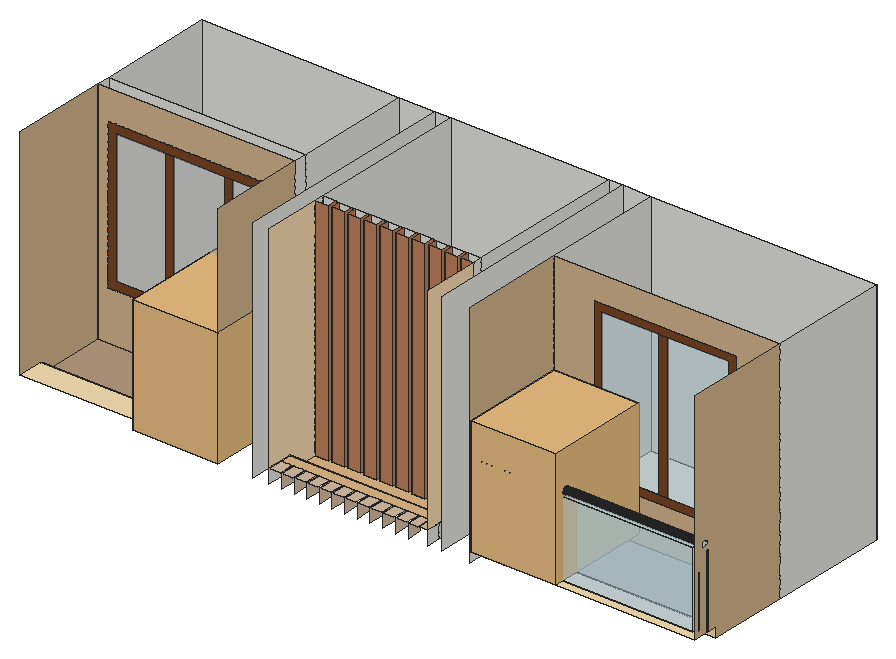
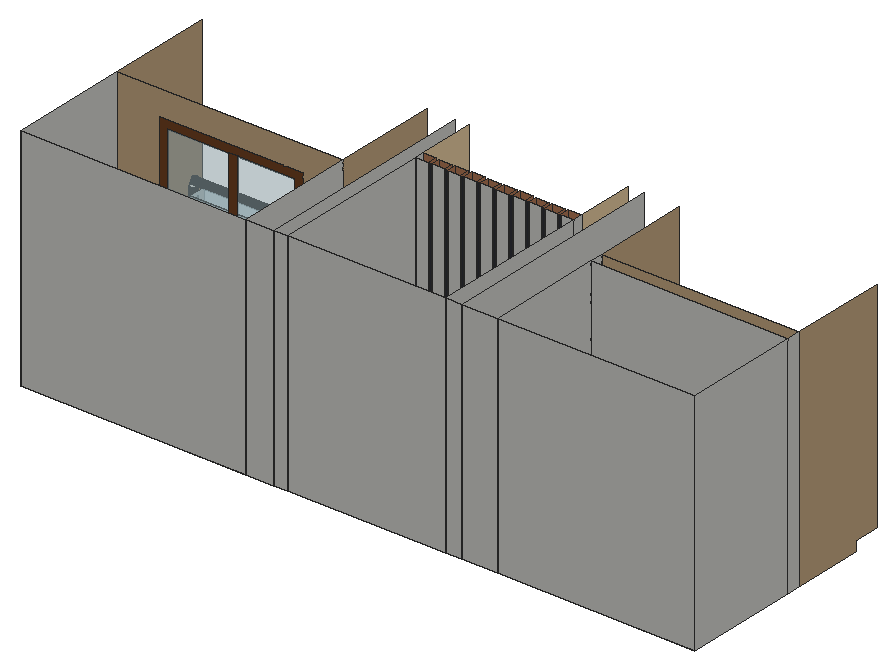
# SketchUp Ruby script. Lengths in inches.
U = 1.inch
M = Sketchup.active_model
def pt(a) = Geom::Point3d.new(a.map { |v| v * U })
def face(e, loops, mat)
  f = e.add_face(loops[0].map { |a| pt(a) })
  loops[1..].each { |l| e.add_face(l.map { |a| pt(a) }).erase! }
  f.material = f.back_material = mat if mat
  f
end
# faces: each face lists its corners as indices into pts; further lists are holes
def faces(e, pts, list, mat = nil) = list.each { |f| face(e, (f[0].is_a?(Array) ? f : [f]).map { |l| l.map { |i| pts[i] } }, mat) }
# xy, xz, yz: faces in a plane at the given z, y or x. An outline is a flat list of corners, or four numbers for a rectangle; further outlines are holes
def ring(l) = l.size == 4 ? [[l[0], l[1]], [l[2], l[1]], [l[2], l[3]], [l[0], l[3]]] : l.each_slice(2).to_a
def flat(e, list, mat, &to3) = list.each { |f| face(e, (f[0].is_a?(Array) ? f : [f]).map { |l| ring(l).map { |u, v| to3.(u, v) } }, mat) }
def xy(e, z, list, mat = nil) = flat(e, list, mat) { |x, y| [x, y, z] }
def xz(e, y, list, mat = nil) = flat(e, list, mat) { |x, z| [x, y, z] }
def yz(e, x, list, mat = nil) = flat(e, list, mat) { |y, z| [x, y, z] }
def lines(e, pts, list) = list.each { |a, b| e.add_line(pt(pts[a]), pt(pts[b])) }
# prism: a flat outline (further loops are holes) pulled along v
def prism(e, loops, v, mat = nil)
  f = face(e, loops, mat); d = Geom::Vector3d.new(v.map { |x| x * U })
  f.pushpull(f.normal.samedirection?(d) ? d.length : -d.length)
end
def box(e, o, s, mat = nil) = prism(e, [[o, [o[0] + s[0], o[1], o[2]], [o[0] + s[0], o[1] + s[1], o[2]], [o[0], o[1] + s[1], o[2]]]], [0, 0, s[2]], mat)
def at(x, y, z, deg = 0) = Geom::Transformation.translation(pt([x, y, z])) * Geom::Transformation.rotation(ORIGIN, Z_AXIS, deg.degrees)
def axes(o, x, y, z) = Geom::Transformation.new([*x, 0, *y, 0, *z, 0, *pt(o).to_a, 1])
def part(name) = M.definitions.add(name)
# library, detail: a bought-in or finely detailed component or shape, given as its bounding box
def library(name, o, s) = part(name).tap { |d| box(d.entities, o, s) }
def detail(e, o, s) = box(e.add_group.entities, o, s)
def put(e, d, t, mat = nil) = e.add_instance(d, t).tap { |i| i.material = mat if mat }
def group(e, t, mat = nil) = e.add_group.tap { |g| g.transformation = t; g.material = mat if mat }.entities
root = M.entities
M.materials.add("[0034_Wheat]").color = [245, 222, 179]
M.materials.add("[0035_Tan]").color = [210, 180, 140]
M.materials.add("[0036_BurlyWood]1").color = [222, 184, 135]
M.materials.add("[Carpet Pattern Leaf Squares Tan]").color = [181, 154, 125]
M.materials.add("[Formica Beige]").color = [247, 219, 174]
M.materials.add("[Formica Laminate Dark]").color = [50, 53, 60]
M.materials.add("[Formica Laminate Light]").color = [213, 189, 164]
M.materials.add("[Tile Travertine 2 inch]").color = [181, 178, 172]
M.materials.add("[Translucent Glass Gray]").color = [191, 191, 191]
M.materials["[Translucent Glass Gray]"].alpha = 0.5
M.materials.add("[Translucent Glass Safety]").color = [204, 235, 244]
M.materials["[Translucent Glass Safety]"].alpha = 0.5
M.materials.add("[Wood Veneer 01]").color = [120, 70, 37]
M.materials.add("[Wood Veneer 02]").color = [190, 128, 91]
c1 = library("chau cay",[-24.34,-109.24,0],[56.46,62.58,79.69])
xy(root,2395.75,[[800.41,467.67,839.27,495.54],[848.6,467.67,887.46,495.54],[896.78,467.67,935.65,495.54],[944.97,467.67,983.83,495.54],[993.16,467.67,1032.02,495.54],
  [1041.35,467.67,1080.21,495.54],[1089.53,467.67,1128.4,495.54],[1137.97,467.67,1176.83,495.54],[1185.96,467.67,1224.82,495.54],[1233.94,467.67,1272.8,495.54],
  [800.41,495.54,1272.8,971.67],[58.44,584.29,646.67,623.89],[1398.32,610.48,2069.85,971.67],[58.44,623.89,646.67,971.67]])
xy(root,2395.75,[[800.41,373.05,1272.8,373.05,1272.8,467.67,1233.94,467.67,1233.94,495.54,1224.82,495.54,1224.82,467.67,1185.96,467.67,1185.96,495.54,1176.83,495.54,1176.83,467.67,1137.97,467.67,1137.97,495.54,1128.4,495.54,1128.4,467.67,1089.53,467.67,1089.53,495.54,1080.21,495.54,1080.21,467.67,1041.35,467.67,1041.35,495.54,1032.02,495.54,1032.02,467.67,993.16,467.67,993.16,495.54,983.83,495.54,983.83,467.67,944.97,467.67,944.97,495.54,935.65,495.54,935.65,467.67,896.78,467.67,896.78,495.54,887.46,495.54,887.46,467.67,848.6,467.67,848.6,495.54,839.27,495.54,839.27,467.67,800.41,467.67]],"[0036_BurlyWood]1")
xy(root,2395.75,[[58.44,373.05,646.67,584.29]],"[Carpet Pattern Leaf Squares Tan]")
xy(root,2395.75,[[1398.32,373.05,2069.85,610.48]],"[Tile Travertine 2 inch]")
xy(root,2425.875,[[1420.76,321.63,2043.52,373.05],[2057.42,331.63,2054.78,331.98,2052.33,333,2050.22,334.61,2048.6,336.72,2047.58,339.18,2047.23,341.82,2047.58,344.46,2048.6,346.91,2050.22,349.02,2052.33,350.64,2054.78,351.66,2057.42,352.01,2060.06,351.66,2062.51,350.64,2064.625,349.02,2066.24,346.91,2067.26,344.46,2067.61,341.82,2067.26,339.18,2066.24,336.72,2064.625,334.61,2062.51,333,2060.06,331.98],[1410.65,336.21,1409.61,336.22,1408.59,336.34,1407.58,336.5625,1406.6,336.89,1405.66,337.32,1404.77,337.84,1403.9375,338.46,1403.17,339.16,1402.49,339.93,1401.89,340.77,1401.38,341.67,1400.97,342.62,1400.66,343.61,1400.45,344.62,1400.35,345.65,1400.36,346.68,1400.48,347.71,1400.71,348.72,1401.03,349.7,1401.46,350.64,1401.99,351.53,1402.6,352.36,1403.3,353.125,1404.08,353.81,1404.92,354.41,1405.82,354.92,1406.77,355.33,1407.75,355.64,1408.77,355.84,1409.79,355.94,1410.83,355.93,1411.85,355.82,1412.86,355.59,1413.84,355.26,1414.78,354.83,1415.67,354.31,1416.51,353.69,1417.27,353,1417.95,352.22,1418.55,351.38,1419.06,350.48,1419.47,349.53,1419.78,348.55,1419.99,347.53,1420.09,346.5,1420.08,345.47,1419.96,344.44,1419.74,343.43,1419.41,342.45,1418.98,341.51,1418.45,340.62,1417.84,339.79,1417.14,339.03,1416.36,338.35,1415.52,337.75,1414.62,337.24,1413.67,336.83,1412.6875,336.52,1411.68,336.31]])
xy(root,2425.875,[[58.44,295.82,646.67,373.05],[1398.32,295.82,2069.85,321.63],[[1398.32,321.63,1420.76,373.05],[1410.65,336.21,1409.61,336.22,1408.59,336.34,1407.58,336.5625,1406.6,336.89,1405.66,337.32,1404.77,337.84,1403.9375,338.46,1403.17,339.16,1402.49,339.93,1401.89,340.77,1401.38,341.67,1400.97,342.62,1400.66,343.61,1400.45,344.62,1400.35,345.65,1400.36,346.68,1400.48,347.71,1400.71,348.72,1401.03,349.7,1401.46,350.64,1401.99,351.53,1402.6,352.36,1403.3,353.125,1404.08,353.81,1404.92,354.41,1405.82,354.92,1406.77,355.33,1407.75,355.64,1408.77,355.84,1409.79,355.94,1410.83,355.93,1411.85,355.82,1412.86,355.59,1413.84,355.26,1414.78,354.83,1415.67,354.31,1416.51,353.69,1417.27,353,1417.95,352.22,1418.55,351.38,1419.06,350.48,1419.47,349.53,1419.78,348.55,1419.99,347.53,1420.09,346.5,1420.08,345.47,1419.96,344.44,1419.74,343.43,1419.41,342.45,1418.98,341.51,1418.45,340.62,1417.84,339.79,1417.14,339.03,1416.36,338.35,1415.52,337.75,1414.62,337.24,1413.67,336.83,1412.6875,336.52,1411.68,336.31]],[[2043.52,321.63,2069.85,373.05],[2057.42,331.63,2054.78,331.98,2052.33,333,2050.22,334.61,2048.6,336.72,2047.58,339.18,2047.23,341.82,2047.58,344.46,2048.6,346.91,2050.22,349.02,2052.33,350.64,2054.78,351.66,2057.42,352.01,2060.06,351.66,2062.51,350.64,2064.625,349.02,2066.24,346.91,2067.26,344.46,2067.61,341.82,2067.26,339.18,2066.24,336.72,2064.625,334.61,2062.51,333,2060.06,331.98]]],"[0034_Wheat]")
xy(root,2437.75,[[800.41,339.19,1272.8,373.05]],"[0036_BurlyWood]1")
xy(root,2437.75,[[800.41,295.82,833.75,339.19],[838.03,295.82,871.37,339.19],[875.66,295.82,909,339.19],[913.28,295.82,946.62,339.19],[950.91,295.82,984.25,339.19],
  [988.53,295.82,1021.87,339.19],[1026.16,295.82,1059.5,339.19],[1063.78,295.82,1097.12,339.19],[1101.41,295.82,1134.75,339.19],[1139.03,295.82,1172.37,339.19],
  [1178.03,295.82,1211.37,339.19],[1215.6,295.82,1244.25,339.19],[1248.93,295.82,1272.8,339.19]],"[Formica Laminate Light]")
xy(root,2648.875,[[1420.76,321.63,2043.52,373.05]],"[Translucent Glass Safety]")
xy(root,2658.625,[[2057.42,331.63,2060.06,331.98,2062.51,333,2064.625,334.61,2066.24,336.72,2067.26,339.18,2067.61,341.82,2067.26,344.46,2066.24,346.91,2064.625,349.02,2062.51,350.64,2060.06,351.66,2057.42,352.01,2054.78,351.66,2052.33,350.64,2050.22,349.02,2048.6,346.91,2047.58,344.46,2047.23,341.82,2047.58,339.18,2048.6,336.72,2050.22,334.61,2052.33,333,2054.78,331.98]])
xy(root,2663.625,[[1410.65,336.21,1411.68,336.31,1412.6875,336.52,1413.67,336.83,1414.62,337.24,1415.52,337.75,1416.36,338.35,1417.14,339.03,1417.84,339.79,1418.45,340.62,1418.98,341.51,1419.41,342.45,1419.74,343.43,1419.96,344.44,1420.08,345.47,1420.09,346.5,1419.99,347.53,1419.78,348.55,1419.47,349.53,1419.06,350.48,1418.55,351.38,1417.95,352.22,1417.27,353,1416.51,353.69,1415.67,354.31,1414.78,354.83,1413.84,355.26,1412.86,355.59,1411.85,355.82,1410.83,355.93,1409.79,355.94,1408.77,355.84,1407.75,355.64,1406.77,355.33,1405.82,354.92,1404.92,354.41,1404.08,353.81,1403.3,353.125,1402.6,352.36,1401.99,351.53,1401.46,350.64,1401.03,349.7,1400.71,348.72,1400.48,347.71,1400.36,346.68,1400.35,345.65,1400.45,344.62,1400.66,343.61,1400.97,342.62,1401.38,341.67,1401.89,340.77,1402.49,339.93,1403.17,339.16,1403.9375,338.46,1404.77,337.84,1405.66,337.32,1406.6,336.89,1407.58,336.5625,1408.59,336.34,1409.61,336.22]])
xz(root,321.63,[[1420.76,2425.875,2043.52,2648.875]],"[Translucent Glass Safety]")
xz(root,373.05,[[58.44,2395.75,646.67,2425.875],[1398.32,2395.75,2069.85,2425.875]],"[0034_Wheat]")
xz(root,373.05,[[800.41,2395.75,1272.8,2437.75]],"[0036_BurlyWood]1")
xz(root,373.05,[[1420.76,2425.875,2043.52,2648.875]],"[Translucent Glass Safety]")
xz(root,467.67,[[800.41,2395.75,839.27,3076.3125],[848.6,2395.75,887.46,3076.3125],[896.78,2395.75,935.65,3076.3125],[944.97,2395.75,983.83,3076.3125],[993.16,2395.75,1032.02,3076.3125],
  [1041.35,2395.75,1080.21,3076.3125],[1089.53,2395.75,1128.4,3076.3125],[1137.97,2395.75,1176.83,3076.3125],[1185.96,2395.75,1224.82,3076.3125],[1233.94,2395.75,1272.8,3076.3125]],"[Wood Veneer 02]")
xz(root,495.54,[[800.41,2395.75,839.27,3076.3125],[848.6,2395.75,887.46,3076.3125],[896.78,2395.75,935.65,3076.3125],[944.97,2395.75,983.83,3076.3125],[993.16,2395.75,1032.02,3076.3125],
  [1041.35,2395.75,1080.21,3076.3125],[1089.53,2395.75,1128.4,3076.3125],[1137.97,2395.75,1176.83,3076.3125],[1185.96,2395.75,1224.82,3076.3125],[1233.94,2395.75,1272.8,3076.3125]])
xz(root,495.54,[[839.27,2395.75,848.6,3076.3125],[887.46,2395.75,896.78,3076.3125],[935.65,2395.75,944.97,3076.3125],[983.83,2395.75,993.16,3076.3125],[1032.02,2395.75,1041.35,3076.3125],
  [1080.21,2395.75,1089.53,3076.3125],[1128.4,2395.75,1137.97,3076.3125],[1176.83,2395.75,1185.96,3076.3125],[1224.82,2395.75,1233.94,3076.3125]],"[Formica Laminate Dark]")
xz(root,584.29,[[[58.44,2395.75,646.67,3076.3125],[89.43,2543.37,617.99,2987.5]]],"[0035_Tan]")
xz(root,584.29,[[114.57,2568.51,260.42,2962.36],[284.1,2568.51,438.79,2962.36],[462.47,2568.51,592.86,2962.36]],"[Translucent Glass Gray]")
xz(root,584.29,[[[89.43,2543.37,617.99,2987.5],[114.57,2568.51,592.86,2962.36]],[260.42,2568.51,284.1,2962.36],[438.79,2568.51,462.47,2962.36]],"[Wood Veneer 01]")
xz(root,610.48,[[[1398.32,2395.75,2069.85,3076.3125],[1515.62,2523,1942.12,3001.19]]],"[0035_Tan]")
xz(root,610.48,[[1539.34,2546.72,1709.53,2977.47],[1737.2,2546.72,1918.4,2977.47]],"[Translucent Glass Safety]")
xz(root,610.48,[[[1515.62,2523,1942.12,3001.19],[1539.34,2546.72,1918.4,2977.47]],[1709.53,2546.72,1737.2,2977.47]],"[Wood Veneer 01]")
xz(root,623.89,[[58.44,2395.75,646.67,3076.3125]])
xz(root,971.67,[[58.44,2395.75,646.67,3076.3125],[646.67,2395.75,752.97,3076.3125],[752.97,2395.75,800.41,3076.3125],[800.41,2395.75,1272.8,3076.3125],[1272.8,2395.75,1313.62,3076.3125],
  [1313.62,2395.75,1398.32,3076.3125],[1398.32,2395.75,2069.85,3076.3125]])
yz(root,58.44,[[584.29,2395.75,623.89,3076.3125],[623.89,2395.75,971.67,3076.3125]])
yz(root,58.44,[[373.05,2395.75,584.29,2395.75,584.29,3076.3125,295.82,3076.3125,295.82,2425.875,373.05,2425.875]],"[0035_Tan]")
yz(root,646.67,[[295.82,2395.75,373.05,2425.875],[584.29,2395.75,623.89,3076.3125],[623.89,2395.75,971.67,3076.3125]])
yz(root,646.67,[[373.05,2395.75,373.05,2425.875,295.82,2425.875,295.82,3076.3125,584.29,3076.3125,584.29,2395.75]],"[0035_Tan]")
yz(root,752.97,[[295.82,2395.75,971.67,3076.3125]])
yz(root,800.41,[[295.82,2395.75,339.19,2437.75],[339.19,2395.75,373.05,2437.75],[467.67,2395.75,495.54,3076.3125],[495.54,2395.75,971.67,3076.3125]])
yz(root,800.41,[[373.05,2395.75,467.67,2395.75,467.67,3076.3125,295.82,3076.3125,295.82,2437.75,373.05,2437.75]],"[Formica Beige]")
yz(root,838.03,[[295.82,2395.75,339.19,2437.75]],"[Formica Laminate Light]")
yz(root,839.27,[[467.67,2395.75,495.54,3076.3125]],"[Wood Veneer 02]")
yz(root,848.6,[[467.67,2395.75,495.54,3076.3125]],"[Wood Veneer 02]")
yz(root,875.66,[[295.82,2395.75,339.19,2437.75]],"[Formica Laminate Light]")
yz(root,887.46,[[467.67,2395.75,495.54,3076.3125]],"[Wood Veneer 02]")
yz(root,896.78,[[467.67,2395.75,495.54,3076.3125]],"[Wood Veneer 02]")
yz(root,913.28,[[295.82,2395.75,339.19,2437.75]],"[Formica Laminate Light]")
yz(root,935.65,[[467.67,2395.75,495.54,3076.3125]],"[Wood Veneer 02]")
yz(root,944.97,[[467.67,2395.75,495.54,3076.3125]],"[Wood Veneer 02]")
yz(root,950.91,[[295.82,2395.75,339.19,2437.75]],"[Formica Laminate Light]")
yz(root,983.83,[[467.67,2395.75,495.54,3076.3125]],"[Wood Veneer 02]")
yz(root,988.53,[[295.82,2395.75,339.19,2437.75]],"[Formica Laminate Light]")
yz(root,993.16,[[467.67,2395.75,495.54,3076.3125]],"[Wood Veneer 02]")
yz(root,1026.16,[[295.82,2395.75,339.19,2437.75]],"[Formica Laminate Light]")
yz(root,1032.02,[[467.67,2395.75,495.54,3076.3125]],"[Wood Veneer 02]")
yz(root,1041.35,[[467.67,2395.75,495.54,3076.3125]],"[Wood Veneer 02]")
yz(root,1063.78,[[295.82,2395.75,339.19,2437.75]],"[Formica Laminate Light]")
yz(root,1080.21,[[467.67,2395.75,495.54,3076.3125]],"[Wood Veneer 02]")
yz(root,1089.53,[[467.67,2395.75,495.54,3076.3125]],"[Wood Veneer 02]")
yz(root,1101.41,[[295.82,2395.75,339.19,2437.75]],"[Formica Laminate Light]")
yz(root,1128.4,[[467.67,2395.75,495.54,3076.3125]],"[Wood Veneer 02]")
yz(root,1137.97,[[467.67,2395.75,495.54,3076.3125]],"[Wood Veneer 02]")
yz(root,1139.03,[[295.82,2395.75,339.19,2437.75]],"[Formica Laminate Light]")
yz(root,1176.83,[[467.67,2395.75,495.54,3076.3125]],"[Wood Veneer 02]")
yz(root,1178.03,[[295.82,2395.75,339.19,2437.75]],"[Formica Laminate Light]")
yz(root,1185.96,[[467.67,2395.75,495.54,3076.3125]],"[Wood Veneer 02]")
yz(root,1215.6,[[295.82,2395.75,339.19,2437.75]],"[Formica Laminate Light]")
yz(root,1224.82,[[467.67,2395.75,495.54,3076.3125]],"[Wood Veneer 02]")
yz(root,1233.94,[[467.67,2395.75,495.54,3076.3125]],"[Wood Veneer 02]")
yz(root,1272.8,[[295.82,2395.75,339.19,2437.75],[339.19,2395.75,373.05,2437.75],[467.67,2395.75,495.54,3076.3125],[495.54,2395.75,971.67,3076.3125]])
yz(root,1272.8,[[373.05,2395.75,373.05,2437.75,295.82,2437.75,295.82,3076.3125,467.67,3076.3125,467.67,2395.75]],"[Formica Beige]")
yz(root,1313.62,[[295.82,2395.75,971.67,3076.3125]])
yz(root,1398.32,[[295.82,2395.75,373.05,2425.875],[610.48,2395.75,971.67,3076.3125]])
yz(root,1398.32,[[[373.05,2395.75,610.48,2395.75,610.48,3076.3125,295.82,3076.3125,295.82,2425.875,373.05,2425.875],[329.5,2655.71,328.47,2655.81,327.46,2656.01,326.47,2656.32,325.52,2656.73,324.62,2657.24,323.78,2657.84,323.01,2658.53,322.31,2659.29,321.69,2660.12,321.17,2661.01,320.74,2661.95,320.41,2662.93,320.1875,2663.94,320.07,2664.97,320.06,2666,320.16,2667.03,320.36,2668.04,320.67,2669.03,321.09,2669.98,321.59,2670.875,322.19,2671.72,322.88,2672.49,323.64,2673.19,324.47,2673.81,325.36,2674.33,326.3,2674.76,327.28,2675.09,328.29,2675.3125,329.32,2675.43,330.35,2675.44,331.38,2675.34,332.39,2675.14,333.38,2674.83,334.33,2674.41,335.23,2673.9,336.07,2673.31,336.84,2672.62,337.54,2671.86,338.16,2671.03,338.68,2670.14,339.11,2669.2,339.44,2668.22,339.66,2667.21,339.78,2666.18,339.79,2665.15,339.69,2664.12,339.49,2663.11,339.18,2662.12,338.76,2661.17,338.26,2660.27,337.66,2659.43,336.97,2658.66,336.21,2657.96,335.38,2657.34,334.49,2656.82,333.55,2656.39,332.57,2656.06,331.56,2655.84,330.53,2655.72]]],"[0035_Tan]")
yz(root,1420.76,[[321.63,2425.875,373.05,2648.875]])
yz(root,2043.52,[[321.63,2425.875,373.05,2648.875]])
yz(root,2069.85,[[610.48,2395.75,971.67,3076.3125],[329.5,2655.71,330.53,2655.72,331.56,2655.84,332.57,2656.06,333.55,2656.39,334.49,2656.82,335.38,2657.34,336.21,2657.96,336.97,2658.66,337.66,2659.43,338.26,2660.27,338.76,2661.17,339.18,2662.12,339.49,2663.11,339.69,2664.12,339.79,2665.15,339.78,2666.18,339.66,2667.21,339.44,2668.22,339.11,2669.2,338.68,2670.14,338.16,2671.03,337.54,2671.86,336.84,2672.62,336.07,2673.31,335.23,2673.9,334.33,2674.41,333.38,2674.83,332.39,2675.14,331.38,2675.34,330.35,2675.44,329.32,2675.43,328.29,2675.3125,327.28,2675.09,326.3,2674.76,325.36,2674.33,324.47,2673.81,323.64,2673.19,322.88,2672.49,322.19,2671.72,321.59,2670.875,321.09,2669.98,320.67,2669.03,320.36,2668.04,320.16,2667.03,320.06,2666,320.07,2664.97,320.1875,2663.94,320.41,2662.93,320.74,2661.95,321.17,2661.01,321.69,2660.12,322.31,2659.29,323.01,2658.53,323.78,2657.84,324.62,2657.24,325.52,2656.73,326.47,2656.32,327.46,2656.01,328.47,2655.81]])
yz(root,2069.85,[[[373.05,2395.75,373.05,2425.875,295.82,2425.875,295.82,3076.3125,610.48,3076.3125,610.48,2395.75],[329.5,2655.71,330.53,2655.72,331.56,2655.84,332.57,2656.06,333.55,2656.39,334.49,2656.82,335.38,2657.34,336.21,2657.96,336.97,2658.66,337.66,2659.43,338.26,2660.27,338.76,2661.17,339.18,2662.12,339.49,2663.11,339.69,2664.12,339.79,2665.15,339.78,2666.18,339.66,2667.21,339.44,2668.22,339.11,2669.2,338.68,2670.14,338.16,2671.03,337.54,2671.86,336.84,2672.62,336.07,2673.31,335.23,2673.9,334.33,2674.41,333.38,2674.83,332.39,2675.14,331.38,2675.34,330.35,2675.44,329.32,2675.43,328.29,2675.3125,327.28,2675.09,326.3,2674.76,325.36,2674.33,324.47,2673.81,323.64,2673.19,322.88,2672.49,322.19,2671.72,321.59,2670.875,321.09,2669.98,320.67,2669.03,320.36,2668.04,320.16,2667.03,320.06,2666,320.07,2664.97,320.1875,2663.94,320.41,2662.93,320.74,2661.95,321.17,2661.01,321.69,2660.12,322.31,2659.29,323.01,2658.53,323.78,2657.84,324.62,2657.24,325.52,2656.73,326.47,2656.32,327.46,2656.01,328.47,2655.81]]],"[0035_Tan]")
p = [[2054.78,331.98,2425.875],[2057.42,331.63,2425.875],[2057.42,331.63,2658.625],[2054.78,331.98,2658.625],[2060.06,331.98,2425.875],[2060.06,331.98,2658.625],
  [2052.33,333,2425.875],[2052.33,333,2658.625],[2062.51,333,2425.875],[2062.51,333,2658.625],[2050.22,334.61,2425.875],[2050.22,334.61,2658.625],
  [2064.625,334.61,2425.875],[2064.625,334.61,2658.625],[2048.6,336.72,2425.875],[2048.6,336.72,2658.625],[2066.24,336.72,2425.875],[2066.24,336.72,2658.625],
  [1408.59,336.34,2425.875],[1409.61,336.22,2425.875],[1409.61,336.22,2663.625],[1408.59,336.34,2663.625],[1410.65,336.21,2425.875],[1410.65,336.21,2663.625],
  [1411.68,336.31,2425.875],[1411.68,336.31,2663.625],[1407.58,336.5625,2425.875],[1407.58,336.5625,2663.625],[1412.6875,336.52,2425.875],[1412.6875,336.52,2663.625],
  [1413.67,336.83,2425.875],[1413.67,336.83,2663.625],[1406.6,336.89,2425.875],[1406.6,336.89,2663.625],[2047.58,339.18,2425.875],[2047.58,339.18,2658.625],
  [2067.26,339.18,2425.875],[2067.26,339.18,2658.625],[1414.62,337.24,2425.875],[1414.62,337.24,2663.625],[1405.66,337.32,2425.875],[1405.66,337.32,2663.625],
  [1415.52,337.75,2425.875],[1415.52,337.75,2663.625],[1404.77,337.84,2425.875],[1404.77,337.84,2663.625],[1416.36,338.35,2425.875],[1416.36,338.35,2663.625],
  [1403.9375,338.46,2425.875],[1403.9375,338.46,2663.625],[1417.14,339.03,2425.875],[1417.14,339.03,2663.625],[1403.17,339.16,2425.875],[1403.17,339.16,2663.625],
  [1417.84,339.79,2425.875],[1417.84,339.79,2663.625],[1402.49,339.93,2425.875],[1402.49,339.93,2663.625],[2047.23,341.82,2425.875],[2047.23,341.82,2658.625],
  [2067.61,341.82,2425.875],[2067.61,341.82,2658.625],[1418.45,340.62,2425.875],[1418.45,340.62,2663.625],[1401.89,340.77,2425.875],[1401.89,340.77,2663.625],
  [1418.98,341.51,2425.875],[1418.98,341.51,2663.625],[1401.38,341.67,2425.875],[1401.38,341.67,2663.625],[1419.41,342.45,2425.875],[1419.41,342.45,2663.625],
  [1400.97,342.62,2425.875],[1400.97,342.62,2663.625],[2047.58,344.46,2425.875],[2047.58,344.46,2658.625],[2067.26,344.46,2425.875],[2067.26,344.46,2658.625],
  [1419.74,343.43,2425.875],[1419.74,343.43,2663.625],[1400.66,343.61,2425.875],[1400.66,343.61,2663.625],[1419.96,344.44,2425.875],[1419.96,344.44,2663.625],
  [1400.45,344.62,2425.875],[1400.45,344.62,2663.625],[1420.08,345.47,2425.875],[1420.08,345.47,2663.625],[2048.6,346.91,2425.875],[2048.6,346.91,2658.625],
  [2066.24,346.91,2425.875],[2066.24,346.91,2658.625],[1400.35,345.65,2425.875],[1400.35,345.65,2663.625],[1420.09,346.5,2425.875],[1420.09,346.5,2663.625],
  [1400.36,346.68,2425.875],[1400.36,346.68,2663.625],[1419.99,347.53,2425.875],[1419.99,347.53,2663.625],[1400.48,347.71,2425.875],[1400.48,347.71,2663.625],
  [2050.22,349.02,2425.875],[2050.22,349.02,2658.625],[2064.625,349.02,2425.875],[2064.625,349.02,2658.625],[1419.78,348.55,2425.875],[1419.78,348.55,2663.625],
  [1400.71,348.72,2425.875],[1400.71,348.72,2663.625],[1419.47,349.53,2425.875],[1419.47,349.53,2663.625],[1401.03,349.7,2425.875],[1401.03,349.7,2663.625],
  [2052.33,350.64,2425.875],[2052.33,350.64,2658.625],[2062.51,350.64,2425.875],[2062.51,350.64,2658.625],[1419.06,350.48,2425.875],[1419.06,350.48,2663.625],
  [1401.46,350.64,2425.875],[1401.46,350.64,2663.625],[1418.55,351.38,2425.875],[1418.55,351.38,2663.625],[1401.99,351.53,2425.875],[1401.99,351.53,2663.625],
  [2054.78,351.66,2425.875],[2054.78,351.66,2658.625],[2060.06,351.66,2425.875],[2060.06,351.66,2658.625],[1417.95,352.22,2425.875],[1417.95,352.22,2663.625],
  [1402.6,352.36,2425.875],[1402.6,352.36,2663.625],[2057.42,352.01,2425.875],[2057.42,352.01,2658.625],[1417.27,353,2425.875],[1417.27,353,2663.625],
  [1403.3,353.125,2425.875],[1403.3,353.125,2663.625],[1416.51,353.69,2425.875],[1416.51,353.69,2663.625],[1404.08,353.81,2425.875],[1404.08,353.81,2663.625],
  [1415.67,354.31,2425.875],[1415.67,354.31,2663.625],[1404.92,354.41,2425.875],[1404.92,354.41,2663.625],[1414.78,354.83,2425.875],[1414.78,354.83,2663.625],
  [1405.82,354.92,2425.875],[1405.82,354.92,2663.625],[1413.84,355.26,2425.875],[1413.84,355.26,2663.625],[1406.77,355.33,2425.875],[1406.77,355.33,2663.625],
  [1407.75,355.64,2425.875],[1407.75,355.64,2663.625],[1412.86,355.59,2425.875],[1412.86,355.59,2663.625],[1408.77,355.84,2425.875],[1408.77,355.84,2663.625],
  [1411.85,355.82,2425.875],[1411.85,355.82,2663.625],[1409.79,355.94,2425.875],[1409.79,355.94,2663.625],[1410.83,355.93,2425.875],[1410.83,355.93,2663.625],
  [2069.85,329.5,2655.71],[2069.85,328.47,2655.81],[1398.32,328.47,2655.81],[1398.32,329.5,2655.71],[2069.85,330.53,2655.72],[1398.32,330.53,2655.72],
  [2069.85,331.56,2655.84],[1398.32,331.56,2655.84],[2069.85,327.46,2656.01],[1398.32,327.46,2656.01],[2069.85,332.57,2656.06],[1398.32,332.57,2656.06],
  [2069.85,326.47,2656.32],[1398.32,326.47,2656.32],[2069.85,333.55,2656.39],[1398.32,333.55,2656.39],[2069.85,325.52,2656.73],[1398.32,325.52,2656.73],
  [2069.85,334.49,2656.82],[1398.32,334.49,2656.82],[2069.85,324.62,2657.24],[1398.32,324.62,2657.24],[2069.85,335.38,2657.34],[1398.32,335.38,2657.34],
  [2069.85,323.78,2657.84],[1398.32,323.78,2657.84],[2069.85,336.21,2657.96],[1398.32,336.21,2657.96],[2069.85,323.01,2658.53],[1398.32,323.01,2658.53],
  [2069.85,336.97,2658.66],[1398.32,336.97,2658.66],[2069.85,322.31,2659.29],[1398.32,322.31,2659.29],[2069.85,337.66,2659.43],[1398.32,337.66,2659.43],
  [2069.85,321.69,2660.12],[1398.32,321.69,2660.12],[2069.85,338.26,2660.27],[1398.32,338.26,2660.27],[2069.85,321.17,2661.01],[1398.32,321.17,2661.01],
  [2069.85,338.76,2661.17],[1398.32,338.76,2661.17],[2069.85,320.74,2661.95],[1398.32,320.74,2661.95],[2069.85,339.18,2662.12],[1398.32,339.18,2662.12],
  [2069.85,320.41,2662.93],[1398.32,320.41,2662.93],[2069.85,339.49,2663.11],[1398.32,339.49,2663.11],[2069.85,320.1875,2663.94],[1398.32,320.1875,2663.94],
  [2069.85,339.69,2664.12],[1398.32,339.69,2664.12],[2069.85,320.07,2664.97],[1398.32,320.07,2664.97],[2069.85,339.79,2665.15],[1398.32,339.79,2665.15],
  [2069.85,320.06,2666],[1398.32,320.06,2666],[2069.85,339.78,2666.18],[1398.32,339.78,2666.18],[2069.85,320.16,2667.03],[1398.32,320.16,2667.03],
  [2069.85,339.66,2667.21],[1398.32,339.66,2667.21],[2069.85,320.36,2668.04],[1398.32,320.36,2668.04],[2069.85,339.44,2668.22],[1398.32,339.44,2668.22],
  [2069.85,320.67,2669.03],[1398.32,320.67,2669.03],[2069.85,339.11,2669.2],[1398.32,339.11,2669.2],[2069.85,321.09,2669.98],[1398.32,321.09,2669.98],
  [2069.85,338.68,2670.14],[1398.32,338.68,2670.14],[2069.85,321.59,2670.875],[1398.32,321.59,2670.875],[2069.85,338.16,2671.03],[1398.32,338.16,2671.03],
  [2069.85,322.19,2671.72],[1398.32,322.19,2671.72],[2069.85,337.54,2671.86],[1398.32,337.54,2671.86],[2069.85,322.88,2672.49],[1398.32,322.88,2672.49],
  [2069.85,336.84,2672.62],[1398.32,336.84,2672.62],[2069.85,323.64,2673.19],[1398.32,323.64,2673.19],[2069.85,336.07,2673.31],[1398.32,336.07,2673.31],
  [2069.85,324.47,2673.81],[1398.32,324.47,2673.81],[2069.85,335.23,2673.9],[1398.32,335.23,2673.9],[2069.85,325.36,2674.33],[1398.32,325.36,2674.33],
  [2069.85,334.33,2674.41],[1398.32,334.33,2674.41],[2069.85,326.3,2674.76],[1398.32,326.3,2674.76],[2069.85,333.38,2674.83],[1398.32,333.38,2674.83],
  [2069.85,327.28,2675.09],[1398.32,327.28,2675.09],[2069.85,332.39,2675.14],[1398.32,332.39,2675.14],[2069.85,328.29,2675.3125],[1398.32,328.29,2675.3125],
  [2069.85,331.38,2675.34],[1398.32,331.38,2675.34],[2069.85,329.32,2675.43],[1398.32,329.32,2675.43],[2069.85,330.35,2675.44],[1398.32,330.35,2675.44]]
faces(root,p,[[0,1,2,3],[1,4,5,2],[6,0,3,7],[4,8,9,5],[10,6,7,11],[8,12,13,9],[14,10,11,15],[12,16,17,13],
  [18,19,20,21],[19,22,23,20],[22,24,25,23],[26,18,21,27],[24,28,29,25],[28,30,31,29],[32,26,27,33],[34,14,15,35],
  [16,36,37,17],[30,38,39,31],[40,32,33,41],[38,42,43,39],[44,40,41,45],[42,46,47,43],[48,44,45,49],[46,50,51,47],
  [52,48,49,53],[50,54,55,51],[56,52,53,57],[58,34,35,59],[36,60,61,37],[54,62,63,55],[64,56,57,65],[62,66,67,63],
  [68,64,65,69],[66,70,71,67],[72,68,69,73],[74,58,59,75],[60,76,77,61],[70,78,79,71],[80,72,73,81],[78,82,83,79],
  [84,80,81,85],[82,86,87,83],[88,74,75,89],[76,90,91,77],[92,84,85,93],[86,94,95,87],[96,92,93,97],[94,98,99,95],
  [100,96,97,101],[102,88,89,103],[90,104,105,91],[98,106,107,99],[108,100,101,109],[106,110,111,107],[112,108,109,113],[114,102,103,115],
  [104,116,117,105],[110,118,119,111],[120,112,113,121],[118,122,123,119],[124,120,121,125],[126,114,115,127],[116,128,129,117],[122,130,131,123],
  [132,124,125,133],[134,126,127,135],[128,134,135,129],[130,136,137,131],[138,132,133,139],[136,140,141,137],[142,138,139,143],[140,144,145,141],
  [146,142,143,147],[144,148,149,145],[150,146,147,151],[148,152,153,149],[154,150,151,155],[156,154,155,157],[152,158,159,153],[160,156,157,161],
  [158,162,163,159],[164,160,161,165],[162,166,167,163],[166,164,165,167],[168,169,170,171],[172,168,171,173],[174,172,173,175],[169,176,177,170],
  [178,174,175,179],[176,180,181,177],[182,178,179,183],[180,184,185,181],[186,182,183,187],[184,188,189,185],[190,186,187,191],[188,192,193,189],
  [194,190,191,195],[192,196,197,193],[198,194,195,199],[196,200,201,197],[202,198,199,203],[200,204,205,201],[206,202,203,207],[204,208,209,205],
  [210,206,207,211],[208,212,213,209],[214,210,211,215],[212,216,217,213],[218,214,215,219],[216,220,221,217],[222,218,219,223],[220,224,225,221],
  [226,222,223,227],[224,228,229,225],[230,226,227,231],[228,232,233,229],[234,230,231,235],[232,236,237,233],[238,234,235,239],[236,240,241,237],
  [242,238,239,243],[240,244,245,241],[246,242,243,247],[244,248,249,245],[250,246,247,251],[248,252,253,249],[254,250,251,255],[252,256,257,253],
  [258,254,255,259],[256,260,261,257],[262,258,259,263],[260,264,265,261],[266,262,263,267],[264,268,269,265],[270,266,267,271],[268,272,273,269],
  [274,270,271,275],[272,276,277,273],[278,274,275,279],[276,280,281,277],[282,278,279,283],[280,284,285,281],[286,282,283,287],[284,286,287,285]],"[Formica Laminate Dark]")
put(root,c1,axes([502.14,64.16,2395.75],[4.5,0,0],[0,-4.9651,0],[0,0,4.37432]))
put(root,c1,axes([1510.42,64.16,2425.875],[4.5,0,0],[0,-4.9651,0],[0,0,4.37432]))
